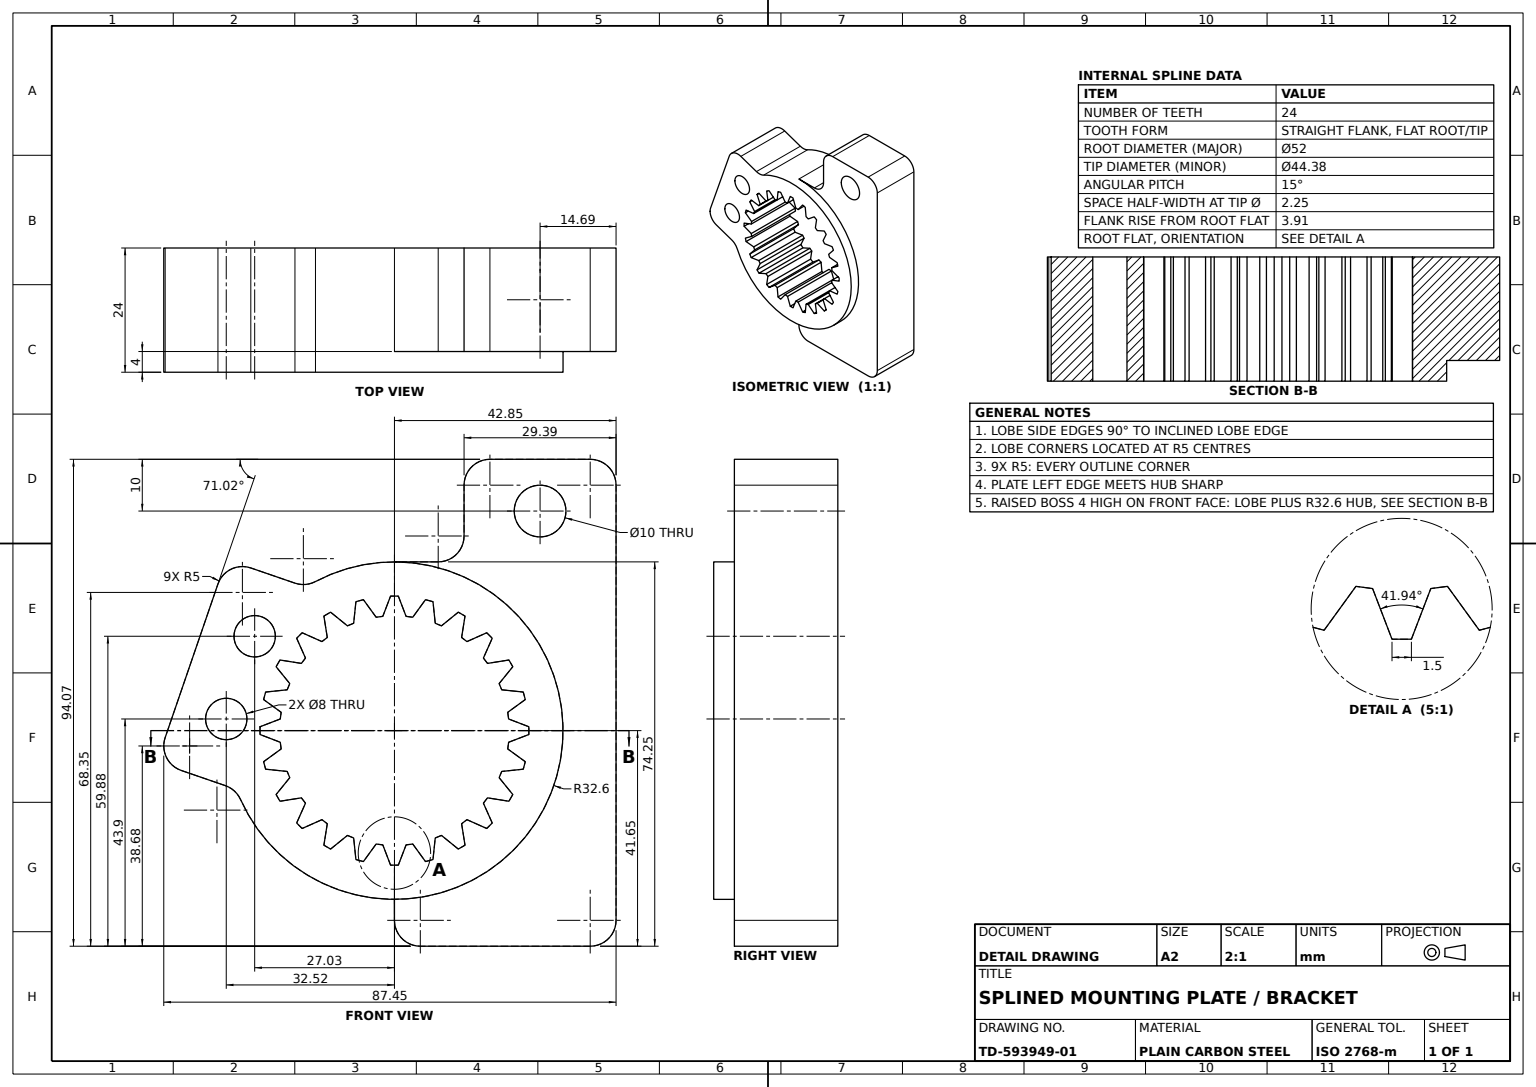
solid
v1 (-2.25,22.075634,0)
v2 (-0.75,25.98918,0)
e1 v1 v2 LINE
v3 (-0.75,25.98918,24)
e2 v3 v2 LINE
v4 (-2.25,22.075634,24)
e3 v3 v4 LINE
e4 v4 v1 LINE
face PLANE(AX(P(-9.339241,3.579582,20),D(-0.933761503,0.357895873,0),D(-0.357895873,-0.933761503,0))) rev [e1 -e2 e3 e4]
v5 (9.08926,20.24306,0)
v6 (7.886928,20.741082,0)
e5 v5 v6 CIRCLE(AX(P(0,0,0),D(0,0,1),D(1,0,0)),22.19)
v7 (9.08926,20.24306,24)
e6 v7 v5 LINE
v8 (7.886928,20.741082,24)
e7 v7 v8 CIRCLE(AX(P(0,0,24),D(0,0,1),D(1,0,0)),22.19)
e8 v8 v6 LINE
face CYL(AX(P(0,0,20),D(0,0,-1),D(-1,0,0)),22.19) rev [-e5 -e6 e7 e8]
v9 (-12.986374,17.99306,24)
v10 (-14.01884,17.20082,24)
e9 v9 v10 CIRCLE(AX(P(0,0,24),D(0,0,1),D(1,0,0)),22.19)
v11 (-14.01884,17.20082,0)
e10 v10 v11 LINE
v12 (-12.986374,17.99306,0)
e11 v12 v11 CIRCLE(AX(P(0,0,0),D(0,0,1),D(1,0,0)),22.19)
e12 v9 v12 LINE
face CYL(AX(P(0,0,20),D(0,0,-1),D(-1,0,0)),22.19) rev [e9 e10 -e11 -e12]
v13 (-17.99306,-12.986374,0)
v14 (-17.20082,-14.01884,0)
e13 v13 v14 CIRCLE(AX(P(0,0,0),D(0,0,1),D(1,0,0)),22.19)
v15 (-17.99306,-12.986374,24)
e14 v15 v13 LINE
v16 (-17.20082,-14.01884,24)
e15 v15 v16 CIRCLE(AX(P(0,0,24),D(0,0,1),D(1,0,0)),22.19)
e16 v16 v14 LINE
face CYL(AX(P(0,0,20),D(0,0,-1),D(-1,0,0)),22.19) rev [-e13 -e14 e15 e16]
v17 (18.907456,17.846796,24)
v18 (18.907456,17.846796,0)
e17 v17 v18 LINE
v19 (17.846796,18.907456,24)
e18 v17 v19 CIRCLE(AX(P(0,0,24),D(0,0,1),D(1,0,0)),26)
v20 (17.846796,18.907456,0)
e19 v19 v20 LINE
e20 v18 v20 CIRCLE(AX(P(0,0,0),D(0,0,1),D(1,0,0)),26)
face CYL(AX(P(0,0,20),D(0,0,-1),D(-1,0,0)),26) rev [-e17 e18 e19 -e20]
v21 (-22.13229,-13.644109,0)
e21 v13 v21 LINE
v22 (-22.13229,-13.644109,24)
e22 v22 v21 LINE
e23 v22 v15 LINE
face PLANE(AX(P(1.569612,-9.877811,20),D(0.156933833,-0.987609119,0),D(0.987609119,0.156933833,0))) rev [e21 -e22 e23 e14]
v23 (18.46,52.42,20)
v24 (13.46,47.42,20)
e24 v23 v24 CIRCLE(AX(P(18.46,47.42,20),D(0,0,1),D(1,0,0)),5)
v25 (18.46,52.42,0)
e25 v23 v25 LINE
v26 (13.46,47.42,0)
e26 v25 v26 CIRCLE(AX(P(18.46,47.42,0),D(0,0,1),D(1,0,0)),5)
e27 v24 v26 LINE
face CYL(AX(P(18.46,47.42,20),D(0,0,-1),D(-1,0,0)),5) [-e24 e25 e26 -e27]
v27 (-17.20082,14.01884,24)
v28 (-17.20082,14.01884,0)
e28 v27 v28 LINE
v29 (-18.907456,17.846796,0)
e29 v28 v29 LINE
v30 (-18.907456,17.846796,24)
e30 v30 v29 LINE
e31 v30 v27 LINE
face PLANE(AX(P(-9.134988,-4.072694,20),D(-0.913339689,-0.407198492,0),D(0.407198492,-0.913339689,0))) rev [e28 e29 -e30 e31]
v31 (13.644109,22.13229,0)
v32 (12.345071,22.88229,0)
e32 v31 v32 CIRCLE(AX(P(0,0,0),D(0,0,1),D(1,0,0)),26)
v33 (13.644109,22.13229,24)
e33 v33 v31 LINE
v34 (12.345071,22.88229,24)
e34 v33 v34 CIRCLE(AX(P(0,0,24),D(0,0,1),D(1,0,0)),26)
e35 v34 v32 LINE
face CYL(AX(P(0,0,20),D(0,0,-1),D(-1,0,0)),26) rev [-e32 -e33 e34 e35]
v35 (17.20082,-14.01884,24)
v36 (17.20082,-14.01884,0)
e36 v35 v36 LINE
v37 (18.907456,-17.846796,0)
e37 v36 v37 LINE
v38 (18.907456,-17.846796,24)
e38 v38 v37 LINE
e39 v38 v35 LINE
face PLANE(AX(P(9.134988,4.072694,20),D(0.913339689,0.407198492,0),D(-0.407198492,0.913339689,0))) rev [e36 e37 -e38 e39]
v39 (3.540261,21.905768,0)
v40 (6.00205,25.297735,0)
e40 v39 v40 LINE
v41 (6.00205,25.297735,24)
e41 v41 v40 LINE
v42 (3.540261,21.905768,24)
e42 v41 v42 LINE
e43 v42 v39 LINE
face PLANE(AX(P(-8.09455,5.874784,20),D(-0.809314083,0.587376127,0),D(-0.587376127,-0.809314083,0))) rev [e40 -e41 e42 e43]
v43 (7.886928,-20.741082,24)
v44 (7.886928,-20.741082,0)
e44 v43 v44 LINE
v45 (9.08926,-20.24306,24)
e45 v43 v45 CIRCLE(AX(P(0,0,24),D(0,0,1),D(1,0,0)),22.19)
v46 (9.08926,-20.24306,0)
e46 v45 v46 LINE
e47 v44 v46 CIRCLE(AX(P(0,0,0),D(0,0,1),D(1,0,0)),22.19)
face CYL(AX(P(0,0,20),D(0,0,-1),D(-1,0,0)),22.19) rev [-e44 e45 e46 -e47]
v47 (24.909506,7.450939,24)
v48 (24.909506,7.450939,0)
e48 v47 v48 LINE
v49 (20.741082,7.886928,24)
e49 v47 v49 LINE
v50 (20.741082,7.886928,0)
e50 v49 v50 LINE
e51 v50 v48 LINE
face PLANE(AX(P(1.040437,9.947478,20),D(0.104025606,0.994574619,0),D(-0.994574619,0.104025606,0))) rev [-e48 e49 e50 e51]
v51 (17.99306,-12.986374,24)
e52 v35 v51 CIRCLE(AX(P(0,0,24),D(0,0,1),D(1,0,0)),22.19)
v52 (17.99306,-12.986374,0)
e53 v51 v52 LINE
e54 v36 v52 CIRCLE(AX(P(0,0,0),D(0,0,1),D(1,0,0)),22.19)
face CYL(AX(P(0,0,20),D(0,0,-1),D(-1,0,0)),22.19) rev [-e36 e52 e53 -e54]
v53 (-34.128801,28.325223,24)
v54 (-34.128801,28.325223,0)
e55 v53 v54 LINE
v55 (-44.331703,-1.339195,0)
e56 v55 v54 LINE
v56 (-44.331703,-1.339195,24)
e57 v56 v55 LINE
e58 v53 v56 LINE
face PLANE(AX(P(-39.230252,13.493014,20),D(-0.945630156,0.32524392,0),D(-0.32524392,-0.945630156,0))) [e55 -e56 -e57 -e58]
v57 (12.345071,-22.88229,24)
v58 (12.345071,-22.88229,0)
e59 v57 v58 LINE
e60 v58 v46 LINE
e61 v45 v57 LINE
face PLANE(AX(P(-6.298229,-7.76963,20),D(-0.629713246,-0.776827669,0),D(0.776827669,-0.629713246,0))) rev [e59 e60 -e46 e61]
v59 (24.909506,-7.450939,24)
v60 (24.909506,-7.450939,0)
e62 v59 v60 LINE
v61 (20.741082,-7.886928,0)
e63 v60 v61 LINE
v62 (20.741082,-7.886928,24)
e64 v62 v61 LINE
e65 v62 v59 LINE
face PLANE(AX(P(1.040437,-9.947478,20),D(0.104025606,-0.994574619,0),D(0.994574619,0.104025606,0))) rev [e62 e63 -e64 e65]
v63 (0.75,-25.98918,24)
v64 (0.75,-25.98918,0)
e66 v63 v64 LINE
v65 (2.25,-22.075634,24)
e67 v63 v65 LINE
v66 (2.25,-22.075634,0)
e68 v65 v66 LINE
e69 v66 v64 LINE
face PLANE(AX(P(9.339241,-3.579582,20),D(0.933761503,-0.357895873,0),D(0.357895873,0.933761503,0))) rev [-e66 e67 e68 e69]
v67 (-22.075634,-2.25,24)
v68 (-22.075634,-2.25,0)
e70 v67 v68 LINE
v69 (-25.98918,-0.75,0)
e71 v68 v69 LINE
v70 (-25.98918,-0.75,24)
e72 v70 v69 LINE
e73 v70 v67 LINE
face PLANE(AX(P(-3.579582,-9.339241,20),D(-0.357895873,-0.933761503,0),D(0.933761503,-0.357895873,0))) rev [e70 e71 -e72 e73]
v71 (-20.741082,7.886928,24)
v72 (-20.741082,7.886928,0)
e74 v71 v72 LINE
v73 (-20.24306,9.08926,0)
e75 v73 v72 CIRCLE(AX(P(0,0,0),D(0,0,1),D(1,0,0)),22.19)
v74 (-20.24306,9.08926,24)
e76 v74 v73 LINE
e77 v74 v71 CIRCLE(AX(P(0,0,24),D(0,0,1),D(1,0,0)),22.19)
face CYL(AX(P(0,0,20),D(0,0,-1),D(-1,0,0)),22.19) rev [e74 -e75 -e76 e77]
v75 (-27.774431,31.427154,24)
v76 (-27.774431,31.427154,0)
e78 v75 v76 LINE
v77 (-19.239147,28.491494,24)
e79 v75 v77 LINE
v78 (-19.239147,28.491494,0)
e80 v77 v78 LINE
e81 v78 v76 LINE
face PLANE(AX(P(6.72767,19.56036,20),D(-0.32524392,-0.945630156,0),D(0.945630156,-0.32524392,0))) rev [-e78 e79 e80 e81]
v79 (33.16,42.42,20)
v80 (33.16,42.42,0)
e82 v79 v80 LINE
v81 (23.16,42.42,0)
e83 v81 v80 CIRCLE(AX(P(28.16,42.42,0),D(0,0,1),D(1,0,0)),5)
v82 (23.16,42.42,20)
e84 v82 v81 LINE
e85 v82 v79 CIRCLE(AX(P(28.16,42.42,20),D(0,0,1),D(1,0,0)),5)
face CYL(AX(P(28.16,42.42,20),D(0,0,-1),D(-1,0,0)),5) rev [e82 -e83 -e84 e85]
v83 (2.25,22.075634,24)
v84 (2.25,22.075634,0)
e86 v83 v84 LINE
v85 (0.75,25.98918,24)
e87 v83 v85 LINE
v86 (0.75,25.98918,0)
e88 v85 v86 LINE
e89 v86 v84 LINE
face PLANE(AX(P(9.339241,3.579582,20),D(0.933761503,0.357895873,0),D(-0.357895873,0.933761503,0))) rev [-e86 e87 e88 e89]
v87 (0,-32.6,0)
v88 (0,-36.65,0)
e90 v87 v88 LINE
v89 (0,-36.65,20)
e91 v89 v88 LINE
v90 (0,-32.6,20)
e92 v90 v89 LINE
e93 v90 v87 LINE
face PLANE(AX(P(0,0,20),D(1,0,0),D(0,0,-1))) rev [e90 -e91 -e92 e93]
v91 (-6.00205,25.297735,24)
v92 (-6.00205,25.297735,0)
e94 v91 v92 LINE
v93 (-7.450939,24.909506,24)
e95 v91 v93 CIRCLE(AX(P(0,0,24),D(0,0,1),D(1,0,0)),26)
v94 (-7.450939,24.909506,0)
e96 v93 v94 LINE
e97 v92 v94 CIRCLE(AX(P(0,0,0),D(0,0,1),D(1,0,0)),26)
face CYL(AX(P(0,0,20),D(0,0,-1),D(-1,0,0)),26) rev [-e94 e95 e96 -e97]
v95 (-17.846796,18.907456,24)
e98 v10 v95 LINE
v96 (-17.846796,18.907456,0)
e99 v95 v96 LINE
e100 v96 v11 LINE
face PLANE(AX(P(4.072694,9.134988,20),D(0.407198492,0.913339689,0),D(-0.913339689,0.407198492,0))) rev [-e10 e98 e99 e100]
v97 (25.98918,-0.75,24)
v98 (25.98918,-0.75,0)
e101 v97 v98 LINE
v99 (25.98918,0.75,24)
e102 v97 v99 CIRCLE(AX(P(0,0,24),D(0,0,1),D(1,0,0)),26)
v100 (25.98918,0.75,0)
e103 v99 v100 LINE
e104 v98 v100 CIRCLE(AX(P(0,0,0),D(0,0,1),D(1,0,0)),26)
face CYL(AX(P(0,0,20),D(0,0,-1),D(-1,0,0)),26) rev [-e101 e102 e103 -e104]
v101 (-22.88229,12.345071,0)
e105 v73 v101 LINE
v102 (-22.88229,12.345071,24)
e106 v102 v101 LINE
e107 v102 v74 LINE
face PLANE(AX(P(-7.76963,-6.298229,20),D(-0.776827669,-0.629713246,0),D(0.629713246,-0.776827669,0))) rev [e76 e105 -e106 e107]
v103 (22.075634,-2.25,24)
v104 (22.075634,-2.25,0)
e108 v103 v104 LINE
e109 v103 v97 LINE
e110 v98 v104 LINE
face PLANE(AX(P(3.579582,-9.339241,20),D(0.357895873,-0.933761503,0),D(0.933761503,0.357895873,0))) rev [-e108 e109 e101 e110]
v105 (7.450939,24.909506,24)
e111 v8 v105 LINE
v106 (7.450939,24.909506,0)
e112 v105 v106 LINE
e113 v106 v6 LINE
face PLANE(AX(P(9.947478,1.040437,20),D(0.994574619,0.104025606,0),D(-0.104025606,0.994574619,0))) rev [e111 e112 e113 -e8]
v107 (-18.907456,-17.846796,24)
v108 (-18.907456,-17.846796,0)
e114 v107 v108 LINE
v109 (-17.846796,-18.907456,24)
e115 v107 v109 CIRCLE(AX(P(0,0,24),D(0,0,1),D(1,0,0)),26)
v110 (-17.846796,-18.907456,0)
e116 v109 v110 LINE
e117 v108 v110 CIRCLE(AX(P(0,0,0),D(0,0,1),D(1,0,0)),26)
face CYL(AX(P(0,0,20),D(0,0,-1),D(-1,0,0)),26) rev [-e114 e115 e116 -e117]
v111 (-22.88229,-12.345071,24)
v112 (-22.88229,-12.345071,0)
e118 v111 v112 LINE
v113 (-20.24306,-9.08926,0)
e119 v112 v113 LINE
v114 (-20.24306,-9.08926,24)
e120 v114 v113 LINE
e121 v114 v111 LINE
face PLANE(AX(P(-7.76963,6.298229,20),D(-0.776827669,0.629713246,0),D(-0.629713246,-0.776827669,0))) rev [e118 e119 -e120 e121]
v115 (-13.644109,22.13229,24)
v116 (-13.644109,22.13229,0)
e122 v115 v116 LINE
e123 v115 v9 LINE
e124 v12 v116 LINE
face PLANE(AX(P(-9.877811,-1.569612,20),D(-0.987609119,-0.156933833,0),D(0.156933833,-0.987609119,0))) rev [-e122 e123 e12 e124]
v117 (37.85,52.42,20)
v118 (37.85,52.42,0)
e125 v117 v118 LINE
v119 (42.85,47.42,20)
e126 v119 v117 CIRCLE(AX(P(37.85,47.42,20),D(0,0,1),D(1,0,0)),5)
v120 (42.85,47.42,0)
e127 v119 v120 LINE
e128 v120 v118 CIRCLE(AX(P(37.85,47.42,0),D(0,0,1),D(1,0,0)),5)
face CYL(AX(P(37.85,47.42,20),D(0,0,-1),D(-1,0,0)),5) [-e125 -e126 e127 e128]
e129 v39 v84 CIRCLE(AX(P(0,0,0),D(0,0,1),D(1,0,0)),22.19)
e130 v42 v83 CIRCLE(AX(P(0,0,24),D(0,0,1),D(1,0,0)),22.19)
face CYL(AX(P(0,0,20),D(0,0,-1),D(-1,0,0)),22.19) rev [-e129 -e43 e130 e86]
v121 (-7.886928,20.741082,0)
e131 v121 v94 LINE
v122 (-7.886928,20.741082,24)
e132 v93 v122 LINE
e133 v122 v121 LINE
face PLANE(AX(P(-9.947478,1.040437,20),D(-0.994574619,0.104025606,0),D(-0.104025606,-0.994574619,0))) rev [e131 -e96 e132 e133]
v123 (-12.345071,22.88229,24)
v124 (-12.345071,22.88229,0)
e134 v123 v124 LINE
v125 (-9.08926,20.24306,0)
e135 v124 v125 LINE
v126 (-9.08926,20.24306,24)
e136 v126 v125 LINE
e137 v126 v123 LINE
face PLANE(AX(P(6.298229,7.76963,20),D(0.629713246,0.776827669,0),D(-0.776827669,0.629713246,0))) rev [e134 e135 -e136 e137]
v127 (-44.603552,-2.965415,0)
v128 (-41.229772,-7.693565,0)
e138 v127 v128 CIRCLE(AX(P(-39.603552,-2.965415,0),D(0,0,1),D(1,0,0)),5)
v129 (-41.229772,-7.693565,24)
e139 v129 v128 LINE
v130 (-44.603552,-2.965415,24)
e140 v130 v129 CIRCLE(AX(P(-39.603552,-2.965415,24),D(0,0,1),D(1,0,0)),5)
e141 v130 v127 LINE
face CYL(AX(P(-39.603552,-2.965415,20),D(0,0,-1),D(-1,0,0)),5) [e138 -e139 -e140 e141]
v131 (17.846796,-18.907456,0)
v132 (14.01884,-17.20082,0)
e142 v131 v132 LINE
v133 (14.01884,-17.20082,24)
e143 v133 v132 LINE
v134 (17.846796,-18.907456,24)
e144 v133 v134 LINE
e145 v134 v131 LINE
face PLANE(AX(P(-4.072694,-9.134988,20),D(-0.407198492,-0.913339689,0),D(0.913339689,-0.407198492,0))) rev [e142 -e143 e144 e145]
v135 (-24.909506,-7.450939,24)
v136 (-20.741082,-7.886928,24)
e146 v135 v136 LINE
v137 (-20.741082,-7.886928,0)
e147 v136 v137 LINE
v138 (-24.909506,-7.450939,0)
e148 v137 v138 LINE
e149 v135 v138 LINE
face PLANE(AX(P(-1.040437,-9.947478,20),D(-0.104025606,-0.994574619,0),D(0.994574619,-0.104025606,0))) rev [e146 e147 e148 -e149]
e150 v85 v3 CIRCLE(AX(P(0,0,24),D(0,0,1),D(1,0,0)),26)
e151 v86 v2 CIRCLE(AX(P(0,0,0),D(0,0,1),D(1,0,0)),26)
face CYL(AX(P(0,0,20),D(0,0,-1),D(-1,0,0)),26) rev [e150 e2 -e151 -e88]
v139 (20.24306,9.08926,24)
e152 v49 v139 CIRCLE(AX(P(0,0,24),D(0,0,1),D(1,0,0)),22.19)
v140 (20.24306,9.08926,0)
e153 v139 v140 LINE
e154 v50 v140 CIRCLE(AX(P(0,0,0),D(0,0,1),D(1,0,0)),22.19)
face CYL(AX(P(0,0,20),D(0,0,-1),D(-1,0,0)),22.19) rev [e152 e153 -e154 -e50]
v141 (0,32.6,20)
v142 (8.46,32.6,20)
e155 v141 v142 LINE
v143 (8.46,32.6,0)
e156 v142 v143 LINE
v144 (0,32.6,0)
e157 v144 v143 LINE
e158 v141 v144 LINE
face PLANE(AX(P(0,32.6,20),D(0,1,0),D(0,0,1))) [e155 e156 -e157 -e158]
v145 (-26,0,24)
v146 (-26,0,0)
e159 v145 v146 LINE
v147 (-25.98918,0.75,0)
e160 v147 v146 CIRCLE(AX(P(0,0,0),D(0,0,1),D(1,0,0)),26)
v148 (-25.98918,0.75,24)
e161 v148 v147 LINE
e162 v148 v145 CIRCLE(AX(P(0,0,24),D(0,0,1),D(1,0,0)),26)
face CYL(AX(P(0,0,20),D(0,0,-1),D(-1,0,0)),26) rev [e159 -e160 -e161 e162]
e163 v56 v130 CIRCLE(AX(P(-39.603552,-2.965415,24),D(0,0,1),D(1,0,0)),5)
e164 v55 v127 CIRCLE(AX(P(-39.603552,-2.965415,0),D(0,0,1),D(1,0,0)),5)
face CYL(AX(P(-39.603552,-2.965415,20),D(0,0,-1),D(-1,0,0)),5) [-e141 -e163 e57 e164]
v149 (3.540261,-21.905768,24)
e165 v65 v149 CIRCLE(AX(P(0,0,24),D(0,0,1),D(1,0,0)),22.19)
v150 (3.540261,-21.905768,0)
e166 v149 v150 LINE
e167 v66 v150 CIRCLE(AX(P(0,0,0),D(0,0,1),D(1,0,0)),22.19)
face CYL(AX(P(0,0,20),D(0,0,-1),D(-1,0,0)),22.19) rev [-e68 e165 e166 -e167]
v151 (-17.99306,12.986374,24)
v152 (-17.99306,12.986374,0)
e168 v151 v152 LINE
v153 (-22.13229,13.644109,24)
e169 v151 v153 LINE
v154 (-22.13229,13.644109,0)
e170 v153 v154 LINE
e171 v154 v152 LINE
face PLANE(AX(P(1.569612,9.877811,20),D(0.156933833,0.987609119,0),D(-0.987609119,0.156933833,0))) rev [-e168 e169 e170 e171]
v155 (7.450939,-24.909506,24)
v156 (7.450939,-24.909506,0)
e172 v155 v156 LINE
v157 (6.00205,-25.297735,0)
e173 v157 v156 CIRCLE(AX(P(0,0,0),D(0,0,1),D(1,0,0)),26)
v158 (6.00205,-25.297735,24)
e174 v158 v157 LINE
e175 v158 v155 CIRCLE(AX(P(0,0,24),D(0,0,1),D(1,0,0)),26)
face CYL(AX(P(0,0,20),D(0,0,-1),D(-1,0,0)),26) rev [e172 -e173 -e174 e175]
v159 (-2.25,-22.075634,24)
v160 (-2.25,-22.075634,0)
e176 v159 v160 LINE
v161 (-3.540261,-21.905768,0)
e177 v161 v160 CIRCLE(AX(P(0,0,0),D(0,0,1),D(1,0,0)),22.19)
v162 (-3.540261,-21.905768,24)
e178 v162 v161 LINE
e179 v162 v159 CIRCLE(AX(P(0,0,24),D(0,0,1),D(1,0,0)),22.19)
face CYL(AX(P(0,0,20),D(0,0,-1),D(-1,0,0)),22.19) rev [e176 -e177 -e178 e179]
v163 (22.88229,12.345071,24)
v164 (22.13229,13.644109,24)
e180 v163 v164 CIRCLE(AX(P(0,0,24),D(0,0,1),D(1,0,0)),26)
v165 (22.13229,13.644109,0)
e181 v164 v165 LINE
v166 (22.88229,12.345071,0)
e182 v166 v165 CIRCLE(AX(P(0,0,0),D(0,0,1),D(1,0,0)),26)
e183 v163 v166 LINE
face CYL(AX(P(0,0,20),D(0,0,-1),D(-1,0,0)),26) rev [e180 e181 -e182 -e183]
v167 (-25.297735,-6.00205,24)
e184 v167 v135 CIRCLE(AX(P(0,0,24),D(0,0,1),D(1,0,0)),26)
v168 (-25.297735,-6.00205,0)
e185 v168 v138 CIRCLE(AX(P(0,0,0),D(0,0,1),D(1,0,0)),26)
e186 v167 v168 LINE
face CYL(AX(P(0,0,20),D(0,0,-1),D(-1,0,0)),26) rev [e184 e149 -e185 -e186]
v169 (-0.75,-25.98918,0)
e187 v169 v64 CIRCLE(AX(P(0,0,0),D(0,0,1),D(1,0,0)),26)
v170 (-0.75,-25.98918,24)
e188 v170 v169 LINE
e189 v170 v63 CIRCLE(AX(P(0,0,24),D(0,0,1),D(1,0,0)),26)
face CYL(AX(P(0,0,20),D(0,0,-1),D(-1,0,0)),26) rev [-e187 -e188 e189 e66]
e190 v112 v21 CIRCLE(AX(P(0,0,0),D(0,0,1),D(1,0,0)),26)
e191 v111 v22 CIRCLE(AX(P(0,0,24),D(0,0,1),D(1,0,0)),26)
face CYL(AX(P(0,0,20),D(0,0,-1),D(-1,0,0)),26) rev [e22 -e190 -e118 e191]
v171 (-6.00205,-25.297735,0)
e192 v161 v171 LINE
v172 (-6.00205,-25.297735,24)
e193 v172 v171 LINE
e194 v172 v162 LINE
face PLANE(AX(P(8.09455,-5.874784,20),D(0.809314083,-0.587376127,0),D(0.587376127,0.809314083,0))) rev [e192 -e193 e194 e178]
e195 v146 v69 CIRCLE(AX(P(0,0,0),D(0,0,1),D(1,0,0)),26)
e196 v145 v70 CIRCLE(AX(P(0,0,24),D(0,0,1),D(1,0,0)),26)
face CYL(AX(P(0,0,20),D(0,0,-1),D(-1,0,0)),26) rev [e72 -e195 -e159 e196]
v173 (17.20082,14.01884,0)
e197 v18 v173 LINE
v174 (17.20082,14.01884,24)
e198 v174 v173 LINE
e199 v174 v17 LINE
face PLANE(AX(P(9.134988,-4.072694,20),D(0.913339689,-0.407198492,0),D(0.407198492,0.913339689,0))) rev [e197 -e198 e199 e17]
v175 (-13.644109,-22.13229,24)
v176 (-13.644109,-22.13229,0)
e200 v175 v176 LINE
v177 (-12.986374,-17.99306,0)
e201 v176 v177 LINE
v178 (-12.986374,-17.99306,24)
e202 v178 v177 LINE
e203 v178 v175 LINE
face PLANE(AX(P(-9.877811,1.569612,20),D(-0.987609119,0.156933833,0),D(-0.156933833,-0.987609119,0))) rev [e200 e201 -e202 e203]
v179 (13.46,37.6,20)
v180 (13.46,37.6,0)
e204 v179 v180 LINE
e205 v24 v179 LINE
e206 v26 v180 LINE
face PLANE(AX(P(13.46,0,20),D(1,0,0),D(0,0,-1))) rev [-e204 -e205 e27 e206]
v181 (12.986374,-17.99306,24)
v182 (12.986374,-17.99306,0)
e207 v181 v182 LINE
e208 v181 v133 CIRCLE(AX(P(0,0,24),D(0,0,1),D(1,0,0)),22.19)
e209 v182 v132 CIRCLE(AX(P(0,0,0),D(0,0,1),D(1,0,0)),22.19)
face CYL(AX(P(0,0,20),D(0,0,-1),D(-1,0,0)),22.19) rev [-e207 e208 e143 -e209]
v183 (-23.025639,18.23115,0)
v184 (-31.025639,18.23115,0)
e210 v183 v184 CIRCLE(AX(P(-27.025639,18.23115,0),D(0,0,1),D(1,0,0)),4)
v185 (-23.025639,18.23115,24)
e211 v185 v183 LINE
v186 (-31.025639,18.23115,24)
e212 v185 v186 CIRCLE(AX(P(-27.025639,18.23115,24),D(0,0,1),D(1,0,0)),4)
e213 v186 v184 LINE
face CYL(AX(P(-27.025639,18.23115,20),D(0,0,-1),D(-1,0,0)),4) rev [-e210 -e211 e212 e213]
v187 (13.644109,-22.13229,24)
e214 v57 v187 CIRCLE(AX(P(0,0,24),D(0,0,1),D(1,0,0)),26)
v188 (13.644109,-22.13229,0)
e215 v187 v188 LINE
e216 v58 v188 CIRCLE(AX(P(0,0,0),D(0,0,1),D(1,0,0)),26)
face CYL(AX(P(0,0,20),D(0,0,-1),D(-1,0,0)),26) rev [e214 e215 -e216 -e59]
v189 (25.297735,-6.00205,0)
e217 v60 v189 CIRCLE(AX(P(0,0,0),D(0,0,1),D(1,0,0)),26)
v190 (25.297735,-6.00205,24)
e218 v59 v190 CIRCLE(AX(P(0,0,24),D(0,0,1),D(1,0,0)),26)
e219 v190 v189 LINE
face CYL(AX(P(0,0,20),D(0,0,-1),D(-1,0,0)),26) rev [-e217 -e62 e218 e219]
v191 (22.075634,2.25,24)
v192 (22.075634,2.25,0)
e220 v191 v192 LINE
e221 v192 v100 LINE
e222 v99 v191 LINE
face PLANE(AX(P(3.579582,9.339241,20),D(0.357895873,0.933761503,0),D(-0.933761503,0.357895873,0))) rev [e220 e221 -e103 e222]
v193 (-22.075634,2.25,0)
e223 v147 v193 LINE
v194 (-22.075634,2.25,24)
e224 v194 v193 LINE
e225 v194 v148 LINE
face PLANE(AX(P(-3.579582,9.339241,20),D(-0.357895873,0.933761503,0),D(-0.933761503,-0.357895873,0))) rev [e161 e223 -e224 e225]
e226 v124 v116 CIRCLE(AX(P(0,0,0),D(0,0,1),D(1,0,0)),26)
e227 v123 v115 CIRCLE(AX(P(0,0,24),D(0,0,1),D(1,0,0)),26)
face CYL(AX(P(0,0,20),D(0,0,-1),D(-1,0,0)),26) rev [-e226 -e134 e227 e122]
e228 v117 v23 LINE
e229 v118 v25 LINE
face PLANE(AX(P(0,52.42,20),D(0,-1,0),D(1,0,0))) rev [-e25 -e228 e125 e229]
v195 (20.24306,-9.08926,24)
v196 (20.24306,-9.08926,0)
e230 v195 v196 LINE
e231 v195 v62 CIRCLE(AX(P(0,0,24),D(0,0,1),D(1,0,0)),22.19)
e232 v196 v61 CIRCLE(AX(P(0,0,0),D(0,0,1),D(1,0,0)),22.19)
face CYL(AX(P(0,0,20),D(0,0,-1),D(-1,0,0)),22.19) rev [-e230 e231 e64 -e232]
e233 v27 v151 CIRCLE(AX(P(0,0,24),D(0,0,1),D(1,0,0)),22.19)
e234 v28 v152 CIRCLE(AX(P(0,0,0),D(0,0,1),D(1,0,0)),22.19)
face CYL(AX(P(0,0,20),D(0,0,-1),D(-1,0,0)),22.19) rev [-e28 e233 e168 -e234]
e235 v182 v188 LINE
e236 v187 v181 LINE
face PLANE(AX(P(9.877811,1.569612,20),D(0.987609119,0.156933833,0),D(-0.156933833,0.987609119,0))) rev [e235 -e215 e236 e207]
e237 v121 v125 CIRCLE(AX(P(0,0,0),D(0,0,1),D(1,0,0)),22.19)
e238 v122 v126 CIRCLE(AX(P(0,0,24),D(0,0,1),D(1,0,0)),22.19)
face CYL(AX(P(0,0,20),D(0,0,-1),D(-1,0,0)),22.19) rev [e136 -e237 -e133 e238]
v197 (-14.01884,-17.20082,0)
e239 v197 v110 LINE
v198 (-14.01884,-17.20082,24)
e240 v109 v198 LINE
e241 v198 v197 LINE
face PLANE(AX(P(4.072694,-9.134988,20),D(0.407198492,-0.913339689,0),D(0.913339689,0.407198492,0))) rev [e239 -e116 e240 e241]
v199 (25.297735,6.00205,0)
e242 v199 v48 CIRCLE(AX(P(0,0,0),D(0,0,1),D(1,0,0)),26)
v200 (25.297735,6.00205,24)
e243 v200 v199 LINE
e244 v200 v47 CIRCLE(AX(P(0,0,24),D(0,0,1),D(1,0,0)),26)
face CYL(AX(P(0,0,20),D(0,0,-1),D(-1,0,0)),26) rev [-e242 -e243 e244 e48]
v201 (12.986374,17.99306,0)
e245 v31 v201 LINE
v202 (12.986374,17.99306,24)
e246 v202 v201 LINE
e247 v202 v33 LINE
face PLANE(AX(P(9.877811,-1.569612,20),D(0.987609119,-0.156933833,0),D(0.156933833,0.987609119,0))) rev [e245 -e246 e247 e33]
e248 v159 v170 LINE
e249 v169 v160 LINE
face PLANE(AX(P(-9.339241,-3.579582,20),D(-0.933761503,-0.357895873,0),D(0.357895873,-0.933761503,0))) rev [e248 e188 e249 -e176]
v203 (21.905768,3.540261,24)
e250 v191 v203 CIRCLE(AX(P(0,0,24),D(0,0,1),D(1,0,0)),22.19)
v204 (21.905768,3.540261,0)
e251 v203 v204 LINE
e252 v192 v204 CIRCLE(AX(P(0,0,0),D(0,0,1),D(1,0,0)),22.19)
face CYL(AX(P(0,0,20),D(0,0,-1),D(-1,0,0)),22.19) rev [-e220 e250 e251 -e252]
v205 (37.85,-41.65,20)
v206 (37.85,-41.65,0)
e253 v205 v206 LINE
v207 (5,-41.65,20)
e254 v207 v205 LINE
v208 (5,-41.65,0)
e255 v207 v208 LINE
e256 v208 v206 LINE
face PLANE(AX(P(0,-41.65,20),D(0,1,0),D(0,0,1))) rev [-e253 -e254 e255 e256]
v209 (22.13229,-13.644109,24)
v210 (22.88229,-12.345071,24)
e257 v209 v210 CIRCLE(AX(P(0,0,24),D(0,0,1),D(1,0,0)),26)
v211 (22.88229,-12.345071,0)
e258 v210 v211 LINE
v212 (22.13229,-13.644109,0)
e259 v212 v211 CIRCLE(AX(P(0,0,0),D(0,0,1),D(1,0,0)),26)
e260 v209 v212 LINE
face CYL(AX(P(0,0,20),D(0,0,-1),D(-1,0,0)),26) rev [e257 e258 -e259 -e260]
e261 v105 v41 CIRCLE(AX(P(0,0,24),D(0,0,1),D(1,0,0)),26)
e262 v106 v40 CIRCLE(AX(P(0,0,0),D(0,0,1),D(1,0,0)),26)
face CYL(AX(P(0,0,20),D(0,0,-1),D(-1,0,0)),26) rev [-e112 e261 e41 -e262]
v213 (14.01884,17.20082,24)
e263 v19 v213 LINE
v214 (14.01884,17.20082,0)
e264 v213 v214 LINE
e265 v214 v20 LINE
face PLANE(AX(P(-4.072694,9.134988,20),D(-0.407198492,0.913339689,0),D(-0.913339689,-0.407198492,0))) rev [-e19 e263 e264 e265]
e266 v213 v202 CIRCLE(AX(P(0,0,24),D(0,0,1),D(1,0,0)),22.19)
e267 v214 v201 CIRCLE(AX(P(0,0,0),D(0,0,1),D(1,0,0)),22.19)
face CYL(AX(P(0,0,20),D(0,0,-1),D(-1,0,0)),22.19) rev [-e264 e266 e246 -e267]
v215 (-24.909506,7.450939,0)
e268 v215 v72 LINE
v216 (-25.297735,6.00205,0)
e269 v215 v216 CIRCLE(AX(P(0,0,0),D(0,0,1),D(1,0,0)),26)
v217 (-21.905768,3.540261,0)
e270 v217 v216 LINE
e271 v217 v193 CIRCLE(AX(P(0,0,0),D(0,0,1),D(1,0,0)),22.19)
v218 (-21.905768,-3.540261,0)
e272 v68 v218 CIRCLE(AX(P(0,0,0),D(0,0,1),D(1,0,0)),22.19)
e273 v168 v218 LINE
e274 v137 v113 CIRCLE(AX(P(0,0,0),D(0,0,1),D(1,0,0)),22.19)
e275 v108 v14 LINE
e276 v197 v177 CIRCLE(AX(P(0,0,0),D(0,0,1),D(1,0,0)),22.19)
v219 (-12.345071,-22.88229,0)
e277 v176 v219 CIRCLE(AX(P(0,0,0),D(0,0,1),D(1,0,0)),26)
v220 (-9.08926,-20.24306,0)
e278 v220 v219 LINE
v221 (-7.886928,-20.741082,0)
e279 v220 v221 CIRCLE(AX(P(0,0,0),D(0,0,1),D(1,0,0)),22.19)
v222 (-7.450939,-24.909506,0)
e280 v222 v221 LINE
e281 v222 v171 CIRCLE(AX(P(0,0,0),D(0,0,1),D(1,0,0)),26)
e282 v157 v150 LINE
e283 v44 v156 LINE
e284 v131 v37 CIRCLE(AX(P(0,0,0),D(0,0,1),D(1,0,0)),26)
e285 v212 v52 LINE
e286 v196 v211 LINE
v223 (21.905768,-3.540261,0)
e287 v223 v189 LINE
e288 v223 v104 CIRCLE(AX(P(0,0,0),D(0,0,1),D(1,0,0)),22.19)
e289 v199 v204 LINE
e290 v166 v140 LINE
v224 (17.99306,12.986374,0)
e291 v224 v165 LINE
e292 v224 v173 CIRCLE(AX(P(0,0,0),D(0,0,1),D(1,0,0)),22.19)
e293 v5 v32 LINE
v225 (-3.540261,21.905768,0)
e294 v1 v225 CIRCLE(AX(P(0,0,0),D(0,0,1),D(1,0,0)),22.19)
e295 v92 v225 LINE
e296 v96 v29 CIRCLE(AX(P(0,0,0),D(0,0,1),D(1,0,0)),26)
e297 v154 v101 CIRCLE(AX(P(0,0,0),D(0,0,1),D(1,0,0)),26)
v226 (-36.522262,2.25,0)
v227 (-28.522262,2.25,0)
e298 v226 v227 CIRCLE(AX(P(-32.522262,2.25,0),D(0,0,1),D(1,0,0)),4)
e299 v227 v226 CIRCLE(AX(P(-32.522262,2.25,0),D(0,0,1),D(1,0,0)),4)
v228 (42.85,-36.65,0)
e300 v228 v120 LINE
e301 v206 v228 CIRCLE(AX(P(37.85,-36.65,0),D(0,0,1),D(1,0,0)),5)
e302 v88 v208 CIRCLE(AX(P(5,-36.65,0),D(0,0,1),D(1,0,0)),5)
v229 (-29.756784,-13.315172,0)
e303 v229 v87 CIRCLE(AX(P(0,0,0),D(0,0,1),D(1,0,0)),32.6)
v230 (-32.694488,-10.629226,0)
e304 v230 v229 CIRCLE(AX(P(-34.320708,-15.357377,0),D(0,0,-1),D(1,0,0)),5)
e305 v230 v128 LINE
e306 v54 v76 CIRCLE(AX(P(-29.40065,26.699003,0),D(0,0,-1),D(1,0,0)),5)
v231 (-15.270783,28.802139,0)
e307 v78 v231 CIRCLE(AX(P(-17.612928,33.219645,0),D(0,0,1),D(1,0,0)),5)
e308 v144 v231 CIRCLE(AX(P(0,0,0),D(0,0,1),D(1,0,0)),32.6)
e309 v143 v180 CIRCLE(AX(P(8.46,37.6,0),D(0,0,1),D(1,0,0)),5)
e310 v184 v183 CIRCLE(AX(P(-27.025639,18.23115,0),D(0,0,1),D(1,0,0)),4)
e311 v80 v81 CIRCLE(AX(P(28.16,42.42,0),D(0,0,1),D(1,0,0)),5)
face PLANE(AX(P(0,0,0),D(0,0,1),D(1,0,0))) rev [-e105 e75 -e268 e269 -e270 e271 -e223 e160 e195 -e71 e272 -e273 e185 -e148 e274 -e119 e190 -e21 e13 -e275 e117 -e239 e276 -e201 e277 -e278 e279 -e280 e281 -e192 e177 -e249 e187 -e69 e167 -e282 e173 -e283 e47 -e60 e216 -e235 e209 -e142 e284 -e37 e54 -e285 e259 -e286 e232 -e63 e217 -e287 e288 -e110 e104 -e221 e252 -e289 e242 -e51 e154 -e290 e182 -e291 e292 -e197 e20 -e265 e267 -e245 e32 -e293 e5 -e113 e262 -e40 e129 -e89 e151 -e1 e294 -e295 e97 -e131 e237 -e135 e226 -e124 e11 -e100 e296 -e29 e234 -e171 e297] [e298 e299] [-e300 -e301 -e256 -e302 -e90 -e303 -e304 e305 -e138 -e164 e56 e306 -e81 e307 -e308 e157 e309 -e206 -e26 -e229 -e128] [e310 e210] [e83 e311]
e312 v186 v185 CIRCLE(AX(P(-27.025639,18.23115,24),D(0,0,1),D(1,0,0)),4)
v232 (-32.694488,-10.629226,24)
e313 v129 v232 LINE
v233 (-29.756784,-13.315172,24)
e314 v233 v232 CIRCLE(AX(P(-34.320708,-15.357377,24),D(0,0,1),D(1,0,0)),5)
v234 (-15.270783,28.802139,24)
e315 v233 v234 CIRCLE(AX(P(0,0,24),D(0,0,1),D(1,0,0)),32.6)
e316 v77 v234 CIRCLE(AX(P(-17.612928,33.219645,24),D(0,0,1),D(1,0,0)),5)
e317 v75 v53 CIRCLE(AX(P(-29.40065,26.699003,24),D(0,0,1),D(1,0,0)),5)
v235 (-36.522262,2.25,24)
v236 (-28.522262,2.25,24)
e318 v235 v236 CIRCLE(AX(P(-32.522262,2.25,24),D(0,0,1),D(1,0,0)),4)
e319 v236 v235 CIRCLE(AX(P(-32.522262,2.25,24),D(0,0,1),D(1,0,0)),4)
v237 (-7.450939,-24.909506,24)
e320 v237 v172 CIRCLE(AX(P(0,0,24),D(0,0,1),D(1,0,0)),26)
v238 (-7.886928,-20.741082,24)
e321 v238 v237 LINE
v239 (-9.08926,-20.24306,24)
e322 v239 v238 CIRCLE(AX(P(0,0,24),D(0,0,1),D(1,0,0)),22.19)
v240 (-12.345071,-22.88229,24)
e323 v240 v239 LINE
e324 v175 v240 CIRCLE(AX(P(0,0,24),D(0,0,1),D(1,0,0)),26)
e325 v198 v178 CIRCLE(AX(P(0,0,24),D(0,0,1),D(1,0,0)),22.19)
e326 v16 v107 LINE
e327 v136 v114 CIRCLE(AX(P(0,0,24),D(0,0,1),D(1,0,0)),22.19)
v241 (-21.905768,-3.540261,24)
e328 v241 v167 LINE
e329 v67 v241 CIRCLE(AX(P(0,0,24),D(0,0,1),D(1,0,0)),22.19)
v242 (-21.905768,3.540261,24)
e330 v242 v194 CIRCLE(AX(P(0,0,24),D(0,0,1),D(1,0,0)),22.19)
v243 (-25.297735,6.00205,24)
e331 v243 v242 LINE
v244 (-24.909506,7.450939,24)
e332 v244 v243 CIRCLE(AX(P(0,0,24),D(0,0,1),D(1,0,0)),26)
e333 v71 v244 LINE
e334 v153 v102 CIRCLE(AX(P(0,0,24),D(0,0,1),D(1,0,0)),26)
e335 v95 v30 CIRCLE(AX(P(0,0,24),D(0,0,1),D(1,0,0)),26)
v245 (-3.540261,21.905768,24)
e336 v245 v91 LINE
e337 v4 v245 CIRCLE(AX(P(0,0,24),D(0,0,1),D(1,0,0)),22.19)
e338 v34 v7 LINE
v246 (17.99306,12.986374,24)
e339 v246 v174 CIRCLE(AX(P(0,0,24),D(0,0,1),D(1,0,0)),22.19)
e340 v164 v246 LINE
e341 v139 v163 LINE
e342 v203 v200 LINE
v247 (21.905768,-3.540261,24)
e343 v247 v103 CIRCLE(AX(P(0,0,24),D(0,0,1),D(1,0,0)),22.19)
e344 v190 v247 LINE
e345 v210 v195 LINE
e346 v51 v209 LINE
e347 v134 v38 CIRCLE(AX(P(0,0,24),D(0,0,1),D(1,0,0)),26)
e348 v155 v43 LINE
e349 v149 v158 LINE
face PLANE(AX(P(-34.320708,-15.357377,24),D(0,0,1),D(1,0,0))) [-e312 -e212] [e163 e140 e313 -e314 e315 -e316 -e79 e317 e58] [-e318 -e319] [-e248 -e179 -e194 -e320 -e321 -e322 -e323 -e324 -e203 -e325 -e240 -e115 -e326 -e15 -e23 -e191 -e121 -e327 -e146 -e184 -e328 -e329 -e73 -e196 -e162 -e225 -e330 -e331 -e332 -e333 -e77 -e107 -e334 -e169 -e233 -e31 -e335 -e98 -e9 -e123 -e227 -e137 -e238 -e132 -e95 -e336 -e337 -e3 -e150 -e87 -e130 -e42 -e261 -e111 -e7 -e338 -e34 -e247 -e266 -e263 -e18 -e199 -e339 -e340 -e180 -e341 -e152 -e49 -e244 -e342 -e250 -e222 -e102 -e109 -e343 -e344 -e218 -e65 -e231 -e345 -e257 -e346 -e52 -e39 -e347 -e144 -e208 -e236 -e214 -e61 -e45 -e348 -e175 -e349 -e165 -e67 -e189]
face PLANE(AX(P(-1.569612,-9.877811,20),D(-0.156933833,-0.987609119,0),D(0.987609119,-0.156933833,0))) rev [e346 e260 e285 -e53]
e350 v245 v225 LINE
face PLANE(AX(P(8.09455,5.874784,20),D(0.809314083,0.587376127,0),D(-0.587376127,0.809314083,0))) rev [e336 e94 e295 -e350]
e351 v234 v231 LINE
e352 v233 v229 LINE
e353 v141 v90 CIRCLE(AX(P(0,0,20),D(0,0,-1),D(1,0,0)),32.6)
face CYL(AX(P(0,0,20),D(0,0,-1),D(-1,0,0)),32.6) [e158 e308 -e351 -e315 e352 e303 -e93 -e353]
e354 v89 v207 CIRCLE(AX(P(5,-36.65,20),D(0,0,1),D(1,0,0)),5)
face CYL(AX(P(5,-36.65,20),D(0,0,-1),D(-1,0,0)),5) [-e255 -e354 e91 e302]
face PLANE(AX(P(-9.134988,4.072694,20),D(-0.913339689,0.407198492,0),D(-0.407198492,-0.913339689,0))) rev [-e16 e326 e114 e275]
face CYL(AX(P(0,0,20),D(0,0,-1),D(-1,0,0)),22.19) rev [-e294 -e4 e337 e350]
face CYL(AX(P(0,0,20),D(0,0,-1),D(-1,0,0)),26) rev [-e284 -e145 e347 e38]
face CYL(AX(P(-29.40065,26.699003,20),D(0,0,-1),D(-1,0,0)),5) [-e55 -e317 e78 -e306]
v248 (42.85,-36.65,20)
e355 v248 v119 LINE
e356 v248 v228 LINE
face PLANE(AX(P(42.85,0,20),D(-1,0,0),D(0,0,1))) rev [e300 -e127 -e355 e356]
face PLANE(AX(P(-8.09455,-5.874784,20),D(-0.809314083,-0.587376127,0),D(0.587376127,-0.809314083,0))) rev [e174 e282 -e166 e349]
e357 v247 v223 LINE
face PLANE(AX(P(5.874784,8.09455,20),D(0.587376127,0.809314083,0),D(-0.809314083,0.587376127,0))) rev [-e219 e344 e357 e287]
e358 v238 v221 LINE
e359 v237 v222 LINE
face PLANE(AX(P(-9.947478,-1.040437,20),D(-0.994574619,-0.104025606,0),D(0.104025606,-0.994574619,0))) rev [-e358 e321 e359 e280]
e360 v236 v227 LINE
e361 v235 v226 LINE
face CYL(AX(P(-32.522262,2.25,20),D(0,0,-1),D(-1,0,0)),4) rev [-e360 e319 e361 -e299]
e362 v242 v217 LINE
face CYL(AX(P(0,0,20),D(0,0,-1),D(-1,0,0)),22.19) rev [e224 -e271 -e362 e330]
e363 v241 v218 LINE
face CYL(AX(P(0,0,20),D(0,0,-1),D(-1,0,0)),22.19) rev [e363 -e272 -e70 e329]
face CYL(AX(P(0,0,20),D(0,0,-1),D(-1,0,0)),22.19) rev [e325 e202 -e276 -e241]
e364 v142 v179 CIRCLE(AX(P(8.46,37.6,20),D(0,0,1),D(1,0,0)),5)
e365 v205 v248 CIRCLE(AX(P(37.85,-36.65,20),D(0,0,1),D(1,0,0)),5)
e366 v79 v82 CIRCLE(AX(P(28.16,42.42,20),D(0,0,1),D(1,0,0)),5)
face PLANE(AX(P(0,0,20),D(0,0,1),D(1,0,0))) [e126 e228 e24 e205 -e364 -e155 e353 e92 e354 e254 e365 e355] [-e366 -e85]
face PLANE(AX(P(9.947478,-1.040437,20),D(0.994574619,-0.104025606,0),D(0.104025606,0.994574619,0))) rev [e348 e44 e283 -e172]
e367 v246 v224 LINE
face CYL(AX(P(0,0,20),D(0,0,-1),D(-1,0,0)),22.19) rev [e339 e198 -e292 -e367]
face PLANE(AX(P(7.76963,-6.298229,20),D(0.776827669,-0.629713246,0),D(0.629713246,0.776827669,0))) rev [e183 e290 -e153 e341]
face PLANE(AX(P(-5.874784,8.09455,20),D(-0.587376127,0.809314083,0),D(-0.809314083,-0.587376127,0))) rev [e273 -e363 e328 e186]
face PLANE(AX(P(7.76963,6.298229,20),D(0.776827669,0.629713246,0),D(-0.629713246,0.776827669,0))) rev [e286 -e258 e345 e230]
face CYL(AX(P(0,0,20),D(0,0,-1),D(-1,0,0)),22.19) rev [e343 e108 -e288 -e357]
e368 v244 v215 LINE
e369 v243 v216 LINE
face CYL(AX(P(0,0,20),D(0,0,-1),D(-1,0,0)),26) rev [-e269 -e368 e332 e369]
face PLANE(AX(P(-6.298229,7.76963,20),D(-0.629713246,0.776827669,0),D(-0.776827669,-0.629713246,0))) rev [e338 e6 e293 -e35]
face CYL(AX(P(0,0,20),D(0,0,-1),D(-1,0,0)),26) rev [e335 e30 -e296 -e99]
face CYL(AX(P(0,0,20),D(0,0,-1),D(-1,0,0)),26) rev [-e170 e334 e106 -e297]
face CYL(AX(P(28.16,42.42,20),D(0,0,-1),D(-1,0,0)),5) rev [e84 -e311 -e82 e366]
e370 v240 v219 LINE
face CYL(AX(P(0,0,20),D(0,0,-1),D(-1,0,0)),26) rev [-e200 e324 e370 -e277]
face CYL(AX(P(-27.025639,18.23115,20),D(0,0,-1),D(-1,0,0)),4) rev [e312 e211 -e310 -e213]
face CYL(AX(P(37.85,-36.65,20),D(0,0,-1),D(-1,0,0)),5) [-e356 -e365 e253 e301]
face PLANE(AX(P(-5.874784,-8.09455,20),D(-0.587376127,-0.809314083,0),D(0.809314083,-0.587376127,0))) rev [e270 -e369 e331 e362]
face PLANE(AX(P(-1.040437,9.947478,20),D(-0.104025606,0.994574619,0),D(-0.994574619,-0.104025606,0))) rev [e268 -e74 e333 e368]
face CYL(AX(P(8.46,37.6,20),D(0,0,-1),D(-1,0,0)),5) rev [-e156 e364 e204 -e309]
e371 v239 v220 LINE
face PLANE(AX(P(6.298229,-7.76963,20),D(0.629713246,-0.776827669,0),D(0.776827669,0.629713246,0))) rev [e371 e278 -e370 e323]
e372 v232 v230 LINE
face PLANE(AX(P(-6.72767,-19.56036,20),D(-0.32524392,-0.945630156,0),D(0.945630156,-0.32524392,0))) [e139 -e305 -e372 -e313]
face CYL(AX(P(-17.612928,33.219645,20),D(0,0,-1),D(-1,0,0)),5) rev [-e307 -e80 e316 e351]
face PLANE(AX(P(5.874784,-8.09455,20),D(0.587376127,-0.809314083,0),D(0.809314083,0.587376127,0))) rev [e289 -e251 e342 e243]
face CYL(AX(P(-32.522262,2.25,20),D(0,0,-1),D(-1,0,0)),4) rev [e360 -e298 -e361 e318]
face CYL(AX(P(0,0,20),D(0,0,-1),D(-1,0,0)),22.19) rev [-e371 e322 e358 -e279]
face PLANE(AX(P(-1.569612,9.877811,20),D(-0.156933833,0.987609119,0),D(-0.987609119,-0.156933833,0))) rev [e291 -e181 e340 e367]
face CYL(AX(P(0,0,20),D(0,0,-1),D(-1,0,0)),22.19) rev [-e147 e327 e120 -e274]
face CYL(AX(P(0,0,20),D(0,0,-1),D(-1,0,0)),26) rev [-e281 -e359 e320 e193]
face CYL(AX(P(-34.320708,-15.357377,20),D(0,0,-1),D(-1,0,0)),5) rev [e314 e372 e304 -e352]
